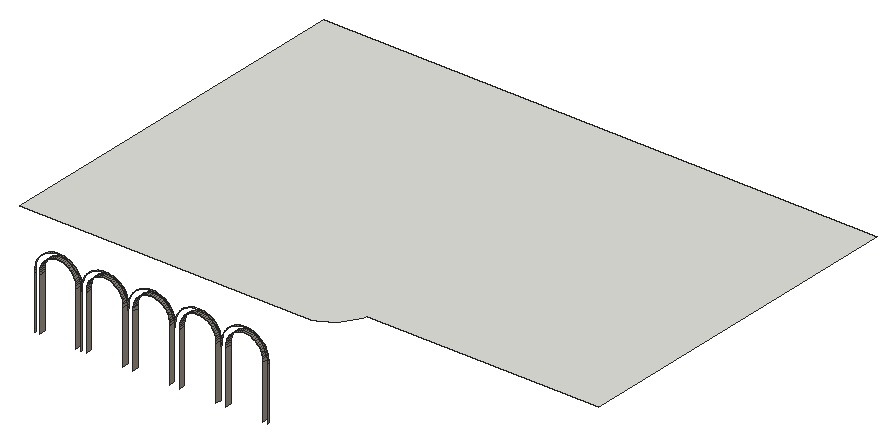
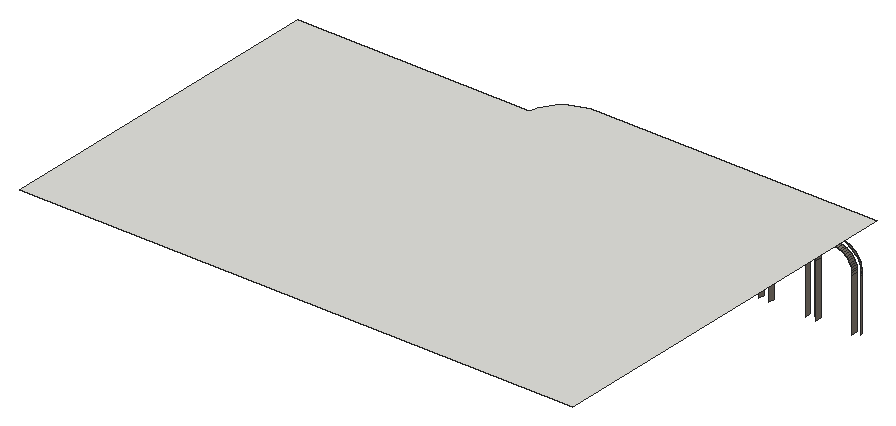
# SketchUp Ruby script. Lengths in inches.
U = 1.inch
M = Sketchup.active_model
def pt(a) = Geom::Point3d.new(a.map { |v| v * U })
def face(e, loops, mat)
  f = e.add_face(loops[0].map { |a| pt(a) })
  loops[1..].each { |l| e.add_face(l.map { |a| pt(a) }).erase! }
  f.material = f.back_material = mat if mat
  f
end
# faces: each face lists its corners as indices into pts; further lists are holes
def faces(e, pts, list, mat = nil) = list.each { |f| face(e, (f[0].is_a?(Array) ? f : [f]).map { |l| l.map { |i| pts[i] } }, mat) }
# xy, xz, yz: faces in a plane at the given z, y or x. An outline is a flat list of corners, or four numbers for a rectangle; further outlines are holes
def ring(l) = l.size == 4 ? [[l[0], l[1]], [l[2], l[1]], [l[2], l[3]], [l[0], l[3]]] : l.each_slice(2).to_a
def flat(e, list, mat, &to3) = list.each { |f| face(e, (f[0].is_a?(Array) ? f : [f]).map { |l| ring(l).map { |u, v| to3.(u, v) } }, mat) }
def xy(e, z, list, mat = nil) = flat(e, list, mat) { |x, y| [x, y, z] }
def xz(e, y, list, mat = nil) = flat(e, list, mat) { |x, z| [x, y, z] }
def yz(e, x, list, mat = nil) = flat(e, list, mat) { |y, z| [x, y, z] }
def lines(e, pts, list) = list.each { |a, b| e.add_line(pt(pts[a]), pt(pts[b])) }
# prism: a flat outline (further loops are holes) pulled along v
def prism(e, loops, v, mat = nil)
  f = face(e, loops, mat); d = Geom::Vector3d.new(v.map { |x| x * U })
  f.pushpull(f.normal.samedirection?(d) ? d.length : -d.length)
end
def box(e, o, s, mat = nil) = prism(e, [[o, [o[0] + s[0], o[1], o[2]], [o[0] + s[0], o[1] + s[1], o[2]], [o[0], o[1] + s[1], o[2]]]], [0, 0, s[2]], mat)
def at(x, y, z, deg = 0) = Geom::Transformation.translation(pt([x, y, z])) * Geom::Transformation.rotation(ORIGIN, Z_AXIS, deg.degrees)
def axes(o, x, y, z) = Geom::Transformation.new([*x, 0, *y, 0, *z, 0, *pt(o).to_a, 1])
def part(name) = M.definitions.add(name)
# library, detail: a bought-in or finely detailed component or shape, given as its bounding box
def library(name, o, s) = part(name).tap { |d| box(d.entities, o, s) }
def detail(e, o, s) = box(e.add_group.entities, o, s)
def put(e, d, t, mat = nil) = e.add_instance(d, t).tap { |i| i.material = mat if mat }
def group(e, t, mat = nil) = e.add_group.tap { |g| g.transformation = t; g.material = mat if mat }.entities
root = M.entities
M.materials.add("Heather_Band").color = [142, 133, 122]
xy(root,1076,[[0,4.77,271.44,4.77,276.08,5.03,280.66,5.83,285.12,7.15,289.4,8.97,293.4375,11.27,297.1875,14.02,300.6,17.18,303.62,20.71,306.22,24.57,308.36,28.69,310.01,33.04,311.15,37.55,311.15,35.95,534.76,35.95,534.76,372.45,0,372.45]])
xz(root,4.77,[[14.55,1023.73,14.55,1026.72,14.51,1026.21],[59.67,1023.73,59.72,1026.21,59.67,1026.72],[104.8,1023.73,104.84,1026.21,104.8,1026.72],[149.92,1023.73,149.96,1026.21,149.92,1026.72],[195.04,1023.73,195.09,1026.21,195.04,1026.72]],"Heather_Band")
yz(root,14.55,[[3.89,972.28,4.77,1023.73],[3.89,1023.73,4.77,1026.72]],"Heather_Band")
yz(root,19.4,[[3.89,972.28,9.67,1023.73],[3.89,1023.73,9.67,1026.5]],"Heather_Band")
yz(root,54.83,[[3.89,972.28,9.67,1023.73],[3.89,1023.73,9.67,1026.5]],"Heather_Band")
yz(root,59.67,[[3.89,972.28,4.02,1023.73],[3.89,1023.73,4.77,1026.72]],"Heather_Band")
yz(root,64.52,[[4.02,972.28,9.67,1023.73],[4.02,1023.73,9.67,1026.5]],"Heather_Band")
yz(root,99.95,[[4.02,972.28,9.67,1023.73],[4.02,1023.73,9.67,1026.5]],"Heather_Band")
yz(root,104.8,[[4.02,1023.73,4.77,1026.72]],"Heather_Band")
yz(root,109.64,[[4.02,972.28,9.67,1023.73],[4.02,1023.73,9.67,1026.5]],"Heather_Band")
yz(root,145.07,[[4.02,972.28,9.67,1023.73],[4.02,1023.73,9.67,1026.5]],"Heather_Band")
yz(root,149.92,[[4.02,1023.73,4.77,1026.72]],"Heather_Band")
yz(root,154.76,[[4.02,972.28,9.67,1023.73],[4.02,1023.73,9.67,1026.5]],"Heather_Band")
yz(root,190.2,[[4.02,972.28,9.67,1023.73],[4.02,1023.73,9.67,1026.5]],"Heather_Band")
yz(root,195.04,[[4.02,1023.73,4.77,1026.72]],"Heather_Band")
yz(root,199.88,[[4.02,972.28,9.67,1023.73],[4.02,1023.73,9.67,1026.5]],"Heather_Band")
yz(root,235.32,[[4.02,972.28,9.67,1023.73],[4.02,1023.73,9.67,1026.5]],"Heather_Band")
yz(root,240.16,[[4.02,972.28,4.77,1023.73],[4.02,1023.73,4.77,1026.72]],"Heather_Band")
p = [[59.72,4.77,1026.21],[59.67,4.77,1023.73],[59.67,4.02,1023.73],[59.72,4.02,1026.21],[104.84,4.77,1026.21],[104.8,4.77,1023.73],
  [104.8,4.02,1023.73],[104.84,4.02,1026.21],[149.96,4.77,1026.21],[149.92,4.77,1023.73],[149.92,4.02,1023.73],[149.96,4.02,1026.21],
  [195.09,4.77,1026.21],[195.04,4.77,1023.73],[195.04,4.02,1023.73],[195.09,4.02,1026.21],[59.67,4.77,1026.72],[59.67,4.02,1026.72],
  [104.8,4.77,1026.72],[104.8,4.02,1026.72],[149.92,4.77,1026.72],[149.92,4.02,1026.72],[195.04,4.77,1026.72],[195.04,4.02,1026.72],
  [19.53,9.67,1027.98],[19.53,3.89,1027.98],[19.4,3.89,1026.5],[19.4,9.67,1026.5],[54.83,9.67,1026.5],[54.83,3.89,1026.5],
  [54.7,3.89,1027.98],[54.7,9.67,1027.98],[64.65,9.67,1027.98],[64.65,4.02,1027.98],[64.52,4.02,1026.5],[64.52,9.67,1026.5],
  [99.95,9.67,1026.5],[99.95,4.02,1026.5],[99.82,4.02,1027.98],[99.82,9.67,1027.98],[109.77,9.67,1027.98],[109.77,4.02,1027.98],
  [109.64,4.02,1026.5],[109.64,9.67,1026.5],[145.07,9.67,1026.5],[145.07,4.02,1026.5],[144.9375,4.02,1027.98],[144.9375,9.67,1027.98],
  [154.9,9.67,1027.98],[154.9,4.02,1027.98],[154.76,4.02,1026.5],[154.76,9.67,1026.5],[190.2,9.67,1026.5],[190.2,4.02,1026.5],
  [190.0625,4.02,1027.98],[190.0625,9.67,1027.98],[200.02,9.67,1027.98],[200.02,4.02,1027.98],[199.88,4.02,1026.5],[199.88,9.67,1026.5],
  [235.32,9.67,1026.5],[235.32,4.02,1026.5],[235.18,4.02,1027.98],[235.18,9.67,1027.98],[14.73,4.77,1028.68],[14.55,4.77,1026.72],
  [14.55,3.89,1026.72],[14.73,3.89,1028.68],[59.5,4.77,1028.68],[59.5,3.89,1028.68],[59.67,3.89,1026.72],[59.85,4.77,1028.68],
  [59.85,4.02,1028.68],[104.62,4.77,1028.68],[104.62,4.02,1028.68],[104.98,4.77,1028.68],[104.98,4.02,1028.68],[149.74,4.77,1028.68],
  [149.74,4.02,1028.68],[150.1,4.77,1028.68],[150.1,4.02,1028.68],[194.86,4.77,1028.68],[194.86,4.02,1028.68],[195.22,4.77,1028.68],
  [195.22,4.02,1028.68],[240.16,4.77,1026.72],[239.98,4.77,1028.68],[239.98,4.02,1028.68],[240.16,4.02,1026.72],[19.92,9.67,1029.88],
  [19.92,3.89,1029.88],[54.31,3.89,1029.88],[54.31,9.67,1029.88],[65.04,9.67,1029.88],[65.04,4.02,1029.88],[99.43,4.02,1029.88],
  [99.43,9.67,1029.88],[110.16,9.67,1029.88],[110.16,4.02,1029.88],[144.55,4.02,1029.88],[144.55,9.67,1029.88],[155.28,9.67,1029.88],
  [155.28,4.02,1029.88],[189.67,4.02,1029.88],[189.67,9.67,1029.88],[200.41,9.67,1029.88],[200.41,4.02,1029.88],[234.8,4.02,1029.88],
  [234.8,9.67,1029.88],[15.23,4.77,1031.11],[15.23,3.89,1031.11],[59,4.77,1031.11],[59,3.89,1031.11],[60.35,4.77,1031.11],
  [60.35,4.02,1031.11],[104.125,4.77,1031.11],[104.125,4.02,1031.11],[105.47,4.77,1031.11],[105.47,4.02,1031.11],[149.25,4.77,1031.11],
  [149.25,4.02,1031.11],[150.59,4.77,1031.11],[150.59,4.02,1031.11],[194.37,4.77,1031.11],[194.37,4.02,1031.11],[195.71,4.77,1031.11],
  [195.71,4.02,1031.11],[239.49,4.77,1031.11],[239.49,4.02,1031.11],[20.51,9.67,1031.74],[20.51,3.89,1031.74],[53.71,3.89,1031.74],
  [53.71,9.67,1031.74],[65.64,9.67,1031.74],[65.64,4.02,1031.74],[98.83,4.02,1031.74],[98.83,9.67,1031.74],[110.76,9.67,1031.74],
  [110.76,4.02,1031.74],[143.96,4.02,1031.74],[143.96,9.67,1031.74],[155.88,9.67,1031.74],[155.88,4.02,1031.74],[189.08,4.02,1031.74],
  [189.08,9.67,1031.74],[201,9.67,1031.74],[201,4.02,1031.74],[234.2,4.02,1031.74],[234.2,9.67,1031.74],[15.98,4.77,1033.47],
  [15.98,3.89,1033.47],[58.24,4.77,1033.47],[58.24,3.89,1033.47],[61.1,4.77,1033.47],[61.1,4.02,1033.47],[103.37,4.77,1033.47],
  [103.37,4.02,1033.47],[106.23,4.77,1033.47],[106.23,4.02,1033.47],[148.49,4.77,1033.47],[148.49,4.02,1033.47],[151.35,4.77,1033.47],
  [151.35,4.02,1033.47],[193.61,4.77,1033.47],[193.61,4.02,1033.47],[196.47,4.77,1033.47],[196.47,4.02,1033.47],[238.73,4.77,1033.47],
  [238.73,4.02,1033.47],[21.31,9.67,1033.52],[21.31,3.89,1033.52],[52.92,3.89,1033.52],[52.92,9.67,1033.52],[66.43,9.67,1033.52],
  [66.43,4.02,1033.52],[98.04,4.02,1033.52],[98.04,9.67,1033.52],[111.55,9.67,1033.52],[111.55,4.02,1033.52],[143.16,4.02,1033.52],
  [143.16,9.67,1033.52],[156.67,9.67,1033.52],[156.67,4.02,1033.52],[188.29,4.02,1033.52],[188.29,9.67,1033.52],[201.79,9.67,1033.52],
  [201.79,4.02,1033.52],[233.41,4.02,1033.52],[233.41,9.67,1033.52],[16.99,4.77,1035.73],[16.99,3.89,1035.73],[22.29,9.67,1035.2],
  [22.29,3.89,1035.2],[51.9375,3.89,1035.2],[51.9375,9.67,1035.2],[57.23,4.77,1035.73],[57.23,3.89,1035.73],[62.11,4.77,1035.73],
  [62.11,4.02,1035.73],[67.41,9.67,1035.2],[67.41,4.02,1035.2],[97.06,4.02,1035.2],[97.06,9.67,1035.2],[102.36,4.77,1035.73],
  [102.36,4.02,1035.73],[107.24,4.77,1035.73],[107.24,4.02,1035.73],[112.53,9.67,1035.2],[112.53,4.02,1035.2],[142.18,4.02,1035.2],
  [142.18,9.67,1035.2],[147.48,4.77,1035.73],[147.48,4.02,1035.73],[152.36,4.77,1035.73],[152.36,4.02,1035.73],[157.66,9.67,1035.2],
  [157.66,4.02,1035.2],[187.3,4.02,1035.2],[187.3,9.67,1035.2],[192.6,4.77,1035.73],[192.6,4.02,1035.73],[197.48,4.77,1035.73],
  [197.48,4.02,1035.73],[202.78,9.67,1035.2],[202.78,4.02,1035.2],[232.42,4.02,1035.2],[232.42,9.67,1035.2],[237.72,4.77,1035.73],
  [237.72,4.02,1035.73],[23.45,9.67,1036.76],[23.45,3.89,1036.76],[50.77,3.89,1036.76],[50.77,9.67,1036.76],[68.57,9.67,1036.76],
  [68.57,4.02,1036.76],[95.9,4.02,1036.76],[95.9,9.67,1036.76],[113.7,9.67,1036.76],[113.7,4.02,1036.76],[141.02,4.02,1036.76],
  [141.02,9.67,1036.76],[158.82,9.67,1036.76],[158.82,4.02,1036.76],[186.14,4.02,1036.76],[186.14,9.67,1036.76],[203.9375,9.67,1036.76],
  [203.9375,4.02,1036.76],[231.26,4.02,1036.76],[231.26,9.67,1036.76],[18.24,4.77,1037.87],[18.24,3.89,1037.87],[55.98,4.77,1037.87],
  [55.98,3.89,1037.87],[63.37,4.77,1037.87],[63.37,4.02,1037.87],[101.1,4.77,1037.87],[101.1,4.02,1037.87],[108.49,4.77,1037.87],
  [108.49,4.02,1037.87],[146.23,4.77,1037.87],[146.23,4.02,1037.87],[153.61,4.77,1037.87],[153.61,4.02,1037.87],[191.35,4.77,1037.87],
  [191.35,4.02,1037.87],[198.73,4.77,1037.87],[198.73,4.02,1037.87],[236.47,4.77,1037.87],[236.47,4.02,1037.87],[24.78,9.67,1038.18],
  [24.78,3.89,1038.18],[49.45,3.89,1038.18],[49.45,9.67,1038.18],[69.9,9.67,1038.18],[69.9,4.02,1038.18],[94.57,4.02,1038.18],
  [94.57,9.67,1038.18],[115.02,9.67,1038.18],[115.02,4.02,1038.18],[139.69,4.02,1038.18],[139.69,9.67,1038.18],[160.14,9.67,1038.18],
  [160.14,4.02,1038.18],[184.82,4.02,1038.18],[184.82,9.67,1038.18],[205.26,9.67,1038.18],[205.26,4.02,1038.18],[229.9375,4.02,1038.18],
  [229.9375,9.67,1038.18],[19.72,4.77,1039.86],[19.72,3.89,1039.86],[54.5,4.77,1039.86],[54.5,3.89,1039.86],[64.84,4.77,1039.86],
  [64.84,4.02,1039.86],[99.625,4.77,1039.86],[99.625,4.02,1039.86],[109.97,4.77,1039.86],[109.97,4.02,1039.86],[144.75,4.77,1039.86],
  [144.75,4.02,1039.86],[155.09,4.77,1039.86],[155.09,4.02,1039.86],[189.87,4.77,1039.86],[189.87,4.02,1039.86],[200.21,4.77,1039.86],
  [200.21,4.02,1039.86],[234.99,4.77,1039.86],[234.99,4.02,1039.86],[26.25,9.67,1039.46],[26.25,3.89,1039.46],[47.98,3.89,1039.46],
  [47.98,9.67,1039.46],[71.37,9.67,1039.46],[71.37,4.02,1039.46],[93.1,4.02,1039.46],[93.1,9.67,1039.46],[116.49,9.67,1039.46],
  [116.49,4.02,1039.46],[138.22,4.02,1039.46],[138.22,9.67,1039.46],[161.62,9.67,1039.46],[161.62,4.02,1039.46],[183.34,4.02,1039.46],
  [183.34,9.67,1039.46],[206.74,9.67,1039.46],[206.74,4.02,1039.46],[228.46,4.02,1039.46],[228.46,9.67,1039.46],[27.85,9.67,1040.5625],
  [27.85,3.89,1040.5625],[46.37,3.89,1040.5625],[46.37,9.67,1040.5625],[72.98,9.67,1040.5625],[72.98,4.02,1040.5625],[91.49,4.02,1040.5625],
  [91.49,9.67,1040.5625],[118.1,9.67,1040.5625],[118.1,4.02,1040.5625],[136.62,4.02,1040.5625],[136.62,9.67,1040.5625],[163.22,9.67,1040.5625],
  [163.22,4.02,1040.5625],[181.74,4.02,1040.5625],[181.74,9.67,1040.5625],[208.34,9.67,1040.5625],[208.34,4.02,1040.5625],[226.86,4.02,1040.5625],
  [226.86,9.67,1040.5625],[21.41,4.77,1041.68],[21.41,3.89,1041.68],[52.82,4.77,1041.68],[52.82,3.89,1041.68],[66.53,4.77,1041.68],
  [66.53,4.02,1041.68],[97.9375,4.77,1041.68],[97.9375,4.02,1041.68],[111.65,4.77,1041.68],[111.65,4.02,1041.68],[143.0625,4.77,1041.68],
  [143.0625,4.02,1041.68],[156.78,4.77,1041.68],[156.78,4.02,1041.68],[188.18,4.77,1041.68],[188.18,4.02,1041.68],[201.9,4.77,1041.68],
  [201.9,4.02,1041.68],[233.3,4.77,1041.68],[233.3,4.02,1041.68],[29.57,9.67,1041.48],[29.57,3.89,1041.48],[44.66,3.89,1041.48],
  [44.66,9.67,1041.48],[74.69,9.67,1041.48],[74.69,4.02,1041.48],[89.78,4.02,1041.48],[89.78,9.67,1041.48],[119.8125,9.67,1041.48],
  [119.8125,4.02,1041.48],[134.9,4.02,1041.48],[134.9,9.67,1041.48],[164.93,9.67,1041.48],[164.93,4.02,1041.48],[180.02,4.02,1041.48],
  [180.02,9.67,1041.48],[210.06,9.67,1041.48],[210.06,4.02,1041.48],[225.15,4.02,1041.48],[225.15,9.67,1041.48],[31.375,9.67,1042.21],
  [31.375,3.89,1042.21],[42.85,3.89,1042.21],[42.85,9.67,1042.21],[76.5,9.67,1042.21],[76.5,4.02,1042.21],[87.97,4.02,1042.21],
  [87.97,9.67,1042.21],[121.62,9.67,1042.21],[121.62,4.02,1042.21],[133.1,4.02,1042.21],[133.1,9.67,1042.21],[166.74,9.67,1042.21],
  [166.74,4.02,1042.21],[178.22,4.02,1042.21],[178.22,9.67,1042.21],[211.86,9.67,1042.21],[211.86,4.02,1042.21],[223.34,4.02,1042.21],
  [223.34,9.67,1042.21],[23.28,4.77,1043.3],[23.28,3.89,1043.3],[50.94,4.77,1043.3],[50.94,3.89,1043.3],[68.41,4.77,1043.3],
  [68.41,4.02,1043.3],[96.0625,4.77,1043.3],[96.0625,4.02,1043.3],[113.53,4.77,1043.3],[113.53,4.02,1043.3],[141.1875,4.77,1043.3],
  [141.1875,4.02,1043.3],[158.65,4.77,1043.3],[158.65,4.02,1043.3],[186.31,4.77,1043.3],[186.31,4.02,1043.3],[203.77,4.77,1043.3],
  [203.77,4.02,1043.3],[231.43,4.77,1043.3],[231.43,4.02,1043.3],[33.25,9.67,1042.74],[33.25,3.89,1042.74],[40.98,3.89,1042.74],
  [40.98,9.67,1042.74],[78.37,9.67,1042.74],[78.37,4.02,1042.74],[86.1,4.02,1042.74],[86.1,9.67,1042.74],[123.49,9.67,1042.74],
  [123.49,4.02,1042.74],[131.22,4.02,1042.74],[131.22,9.67,1042.74],[168.61,9.67,1042.74],[168.61,4.02,1042.74],[176.34,4.02,1042.74],
  [176.34,9.67,1042.74],[213.74,9.67,1042.74],[213.74,4.02,1042.74],[221.47,4.02,1042.74],[221.47,9.67,1042.74],[35.17,9.67,1043.06],
  [35.17,3.89,1043.06],[39.06,3.89,1043.06],[39.06,9.67,1043.06],[80.29,9.67,1043.06],[80.29,4.02,1043.06],[84.18,4.02,1043.06],
  [84.18,9.67,1043.06],[125.41,9.67,1043.06],[125.41,4.02,1043.06],[129.3,4.02,1043.06],[129.3,9.67,1043.06],[170.53,9.67,1043.06],
  [170.53,4.02,1043.06],[174.42,4.02,1043.06],[174.42,9.67,1043.06],[215.66,9.67,1043.06],[215.66,4.02,1043.06],[219.54,4.02,1043.06],
  [219.54,9.67,1043.06],[37.11,9.67,1043.16],[37.11,3.89,1043.16],[82.24,9.67,1043.16],[82.24,4.02,1043.16],[127.36,9.67,1043.16],
  [127.36,4.02,1043.16],[172.48,9.67,1043.16],[172.48,4.02,1043.16],[217.6,9.67,1043.16],[217.6,4.02,1043.16],[25.33,4.77,1044.7],
  [25.33,3.89,1044.7],[48.9,4.77,1044.7],[48.9,3.89,1044.7],[70.45,4.77,1044.7],[70.45,4.02,1044.7],[94.02,4.77,1044.7],
  [94.02,4.02,1044.7],[115.57,4.77,1044.7],[115.57,4.02,1044.7],[139.14,4.77,1044.7],[139.14,4.02,1044.7],[160.69,4.77,1044.7],
  [160.69,4.02,1044.7],[184.27,4.77,1044.7],[184.27,4.02,1044.7],[205.8125,4.77,1044.7],[205.8125,4.02,1044.7],[229.39,4.77,1044.7],
  [229.39,4.02,1044.7],[27.51,4.77,1045.875],[27.51,3.89,1045.875],[46.72,4.77,1045.875],[46.72,3.89,1045.875],[72.63,4.77,1045.875],
  [72.63,4.02,1045.875],[91.84,4.77,1045.875],[91.84,4.02,1045.875],[117.75,4.77,1045.875],[117.75,4.02,1045.875],[136.96,4.77,1045.875],
  [136.96,4.02,1045.875],[162.875,4.77,1045.875],[162.875,4.02,1045.875],[182.08,4.77,1045.875],[182.08,4.02,1045.875],[208,4.77,1045.875],
  [208,4.02,1045.875],[227.2,4.77,1045.875],[227.2,4.02,1045.875],[29.81,4.77,1046.8],[29.81,3.89,1046.8],[44.42,4.77,1046.8],
  [44.42,3.89,1046.8],[74.93,4.77,1046.8],[74.93,4.02,1046.8],[89.54,4.77,1046.8],[89.54,4.02,1046.8],[120.05,4.77,1046.8],
  [120.05,4.02,1046.8],[134.66,4.77,1046.8],[134.66,4.02,1046.8],[165.17,4.77,1046.8],[165.17,4.02,1046.8],[179.78,4.77,1046.8],
  [179.78,4.02,1046.8],[210.3,4.77,1046.8],[210.3,4.02,1046.8],[224.91,4.77,1046.8],[224.91,4.02,1046.8],[32.19,4.77,1047.47],
  [32.19,3.89,1047.47],[42.03,4.77,1047.47],[42.03,3.89,1047.47],[77.32,4.77,1047.47],[77.32,4.02,1047.47],[87.15,4.77,1047.47],
  [87.15,4.02,1047.47],[122.4375,4.77,1047.47],[122.4375,4.02,1047.47],[132.28,4.77,1047.47],[132.28,4.02,1047.47],[167.56,4.77,1047.47],
  [167.56,4.02,1047.47],[177.4,4.77,1047.47],[177.4,4.02,1047.47],[212.68,4.77,1047.47],[212.68,4.02,1047.47],[222.52,4.77,1047.47],
  [222.52,4.02,1047.47],[34.64,4.77,1047.88],[34.64,3.89,1047.88],[39.59,4.77,1047.88],[39.59,3.89,1047.88],[79.76,4.77,1047.88],
  [79.76,4.02,1047.88],[84.71,4.77,1047.88],[84.71,4.02,1047.88],[124.88,4.77,1047.88],[124.88,4.02,1047.88],[129.83,4.77,1047.88],
  [129.83,4.02,1047.88],[170,4.77,1047.88],[170,4.02,1047.88],[174.95,4.77,1047.88],[174.95,4.02,1047.88],[215.125,4.77,1047.88],
  [215.125,4.02,1047.88],[220.08,4.77,1047.88],[220.08,4.02,1047.88],[37.11,4.77,1048.02],[37.11,3.89,1048.02],[82.24,4.77,1048.02],
  [82.24,4.02,1048.02],[127.36,4.77,1048.02],[127.36,4.02,1048.02],[172.48,4.77,1048.02],[172.48,4.02,1048.02],[217.6,4.77,1048.02],
  [217.6,4.02,1048.02]]
faces(root,p,[[0,1,2,3],[4,5,6,7],[8,9,10,11],[12,13,14,15],[16,0,3,17],[18,4,7,19],[20,8,11,21],[22,12,15,23],
  [24,25,26,27],[28,29,30,31],[32,33,34,35],[36,37,38,39],[40,41,42,43],[44,45,46,47],[48,49,50,51],[52,53,54,55],
  [56,57,58,59],[60,61,62,63],[64,65,66,67],[16,68,69,70,17],[71,16,17,72],[18,73,74,19],[75,18,19,76],[20,77,78,21],
  [79,20,21,80],[22,81,82,23],[83,22,23,84],[85,86,87,88],[89,90,25,24],[31,30,91,92],[93,94,33,32],[39,38,95,96],
  [97,98,41,40],[47,46,99,100],[101,102,49,48],[55,54,103,104],[105,106,57,56],[63,62,107,108],[109,64,67,110],[68,111,112,69],
  [113,71,72,114],[73,115,116,74],[117,75,76,118],[77,119,120,78],[121,79,80,122],[81,123,124,82],[125,83,84,126],[86,127,128,87],
  [129,130,90,89],[92,91,131,132],[133,134,94,93],[96,95,135,136],[137,138,98,97],[100,99,139,140],[141,142,102,101],[104,103,143,144],
  [145,146,106,105],[108,107,147,148],[149,109,110,150],[111,151,152,112],[153,113,114,154],[115,155,156,116],[157,117,118,158],[119,159,160,120],
  [161,121,122,162],[123,163,164,124],[165,125,126,166],[127,167,168,128],[169,170,130,129],[132,131,171,172],[173,174,134,133],[136,135,175,176],
  [177,178,138,137],[140,139,179,180],[181,182,142,141],[144,143,183,184],[185,186,146,145],[148,147,187,188],[189,149,150,190],[191,192,170,169],
  [172,171,193,194],[151,195,196,152],[197,153,154,198],[199,200,174,173],[176,175,201,202],[155,203,204,156],[205,157,158,206],[207,208,178,177],
  [180,179,209,210],[159,211,212,160],[213,161,162,214],[215,216,182,181],[184,183,217,218],[163,219,220,164],[221,165,166,222],[223,224,186,185],
  [188,187,225,226],[167,227,228,168],[229,230,192,191],[194,193,231,232],[233,234,200,199],[202,201,235,236],[237,238,208,207],[210,209,239,240],
  [241,242,216,215],[218,217,243,244],[245,246,224,223],[226,225,247,248],[249,189,190,250],[195,251,252,196],[253,197,198,254],[203,255,256,204],
  [257,205,206,258],[211,259,260,212],[261,213,214,262],[219,263,264,220],[265,221,222,266],[227,267,268,228],[269,270,230,229],[232,231,271,272],
  [273,274,234,233],[236,235,275,276],[277,278,238,237],[240,239,279,280],[281,282,242,241],[244,243,283,284],[285,286,246,245],[248,247,287,288],
  [289,249,250,290],[251,291,292,252],[293,253,254,294],[255,295,296,256],[297,257,258,298],[259,299,300,260],[301,261,262,302],[263,303,304,264],
  [305,265,266,306],[267,307,308,268],[309,310,270,269],[272,271,311,312],[313,314,274,273],[276,275,315,316],[317,318,278,277],[280,279,319,320],
  [321,322,282,281],[284,283,323,324],[325,326,286,285],[288,287,327,328],[329,330,310,309],[312,311,331,332],[333,334,314,313],[316,315,335,336],
  [337,338,318,317],[320,319,339,340],[341,342,322,321],[324,323,343,344],[345,346,326,325],[328,327,347,348],[349,289,290,350],[291,351,352,292],
  [353,293,294,354],[295,355,356,296],[357,297,298,358],[299,359,360,300],[361,301,302,362],[303,363,364,304],[365,305,306,366],[307,367,368,308],
  [369,370,330,329],[332,331,371,372],[373,374,334,333],[336,335,375,376],[377,378,338,337],[340,339,379,380],[381,382,342,341],[344,343,383,384],
  [385,386,346,345],[348,347,387,388],[389,390,370,369],[372,371,391,392],[393,394,374,373],[376,375,395,396],[397,398,378,377],[380,379,399,400],
  [401,402,382,381],[384,383,403,404],[405,406,386,385],[388,387,407,408],[409,349,350,410],[351,411,412,352],[413,353,354,414],[355,415,416,356],
  [417,357,358,418],[359,419,420,360],[421,361,362,422],[363,423,424,364],[425,365,366,426],[367,427,428,368],[429,430,390,389],[392,391,431,432],
  [433,434,394,393],[396,395,435,436],[437,438,398,397],[400,399,439,440],[441,442,402,401],[404,403,443,444],[445,446,406,405],[408,407,447,448],
  [449,450,430,429],[432,431,451,452],[453,454,434,433],[436,435,455,456],[457,458,438,437],[440,439,459,460],[461,462,442,441],[444,443,463,464],
  [465,466,446,445],[448,447,467,468],[469,470,450,449],[452,451,470,469],[471,472,454,453],[456,455,472,471],[473,474,458,457],[460,459,474,473],
  [475,476,462,461],[464,463,476,475],[477,478,466,465],[468,467,478,477],[479,409,410,480],[411,481,482,412],[483,413,414,484],[415,485,486,416],
  [487,417,418,488],[419,489,490,420],[491,421,422,492],[423,493,494,424],[495,425,426,496],[427,497,498,428],[499,479,480,500],[481,501,502,482],
  [503,483,484,504],[485,505,506,486],[507,487,488,508],[489,509,510,490],[511,491,492,512],[493,513,514,494],[515,495,496,516],[497,517,518,498],
  [519,499,500,520],[501,521,522,502],[523,503,504,524],[505,525,526,506],[527,507,508,528],[509,529,530,510],[531,511,512,532],[513,533,534,514],
  [535,515,516,536],[517,537,538,518],[539,519,520,540],[521,541,542,522],[543,523,524,544],[525,545,546,526],[547,527,528,548],[529,549,550,530],
  [551,531,532,552],[533,553,554,534],[555,535,536,556],[537,557,558,538],[559,539,540,560],[541,561,562,542],[563,543,544,564],[545,565,566,546],
  [567,547,548,568],[549,569,570,550],[571,551,552,572],[553,573,574,554],[575,555,556,576],[557,577,578,558],[579,559,560,580],[561,579,580,562],
  [581,563,564,582],[565,581,582,566],[583,567,568,584],[569,583,584,570],[585,571,572,586],[573,585,586,574],[587,575,576,588],[577,587,588,578]],"Heather_Band")
